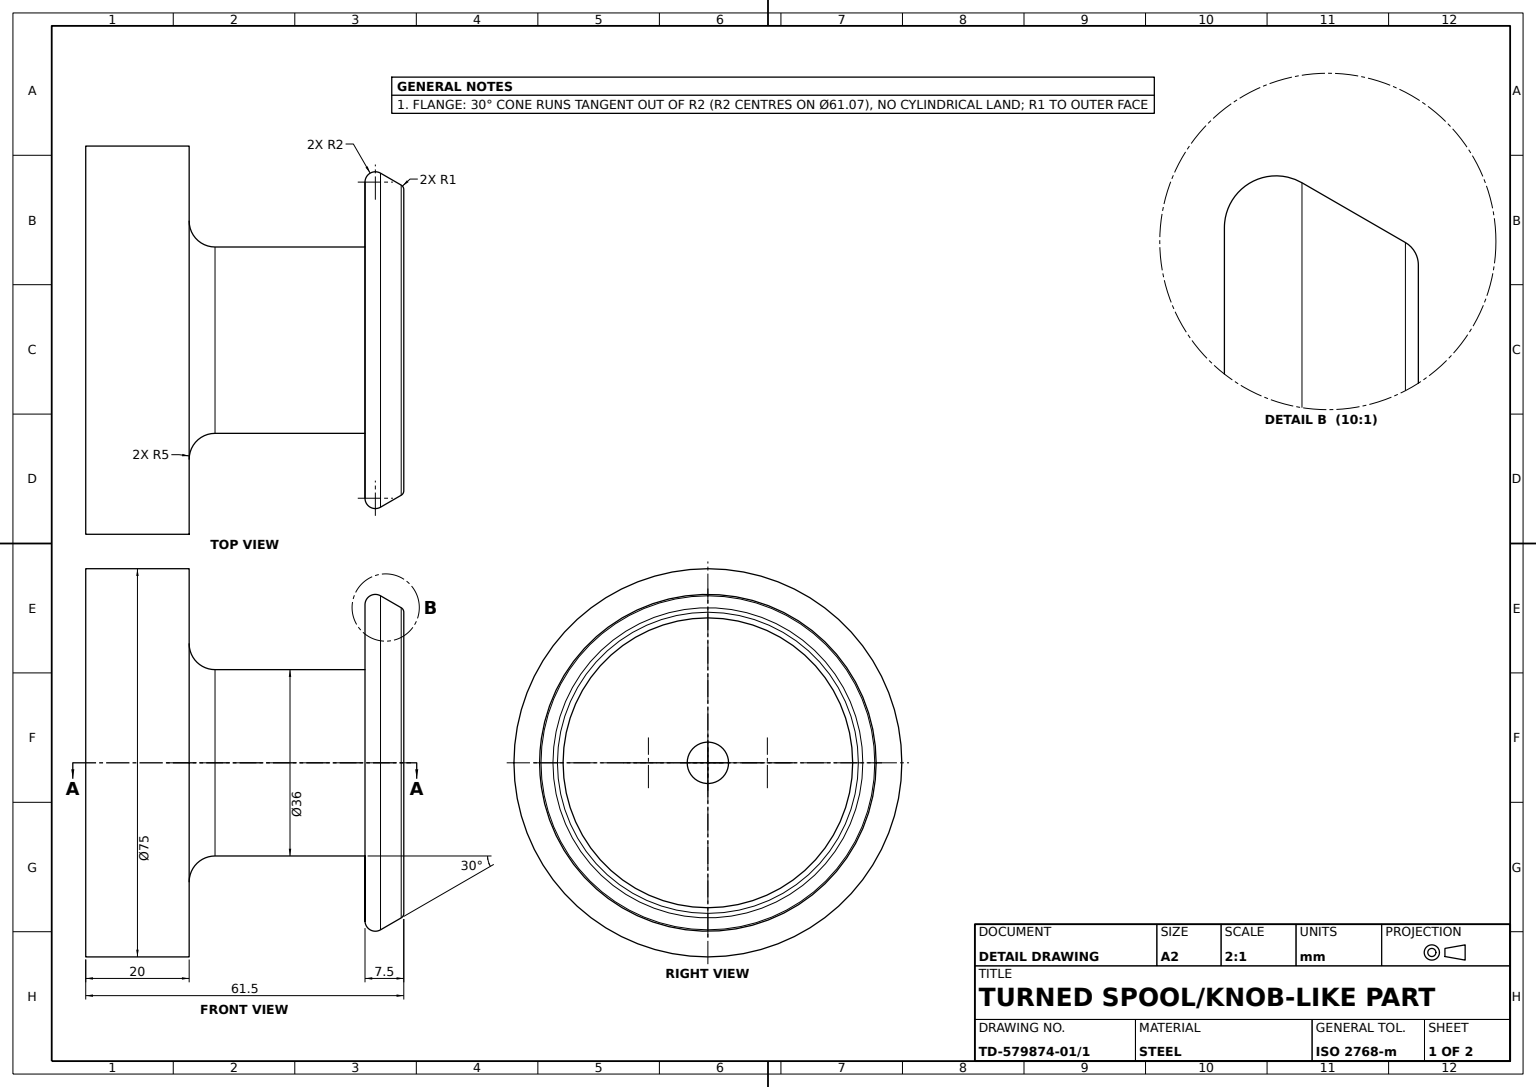
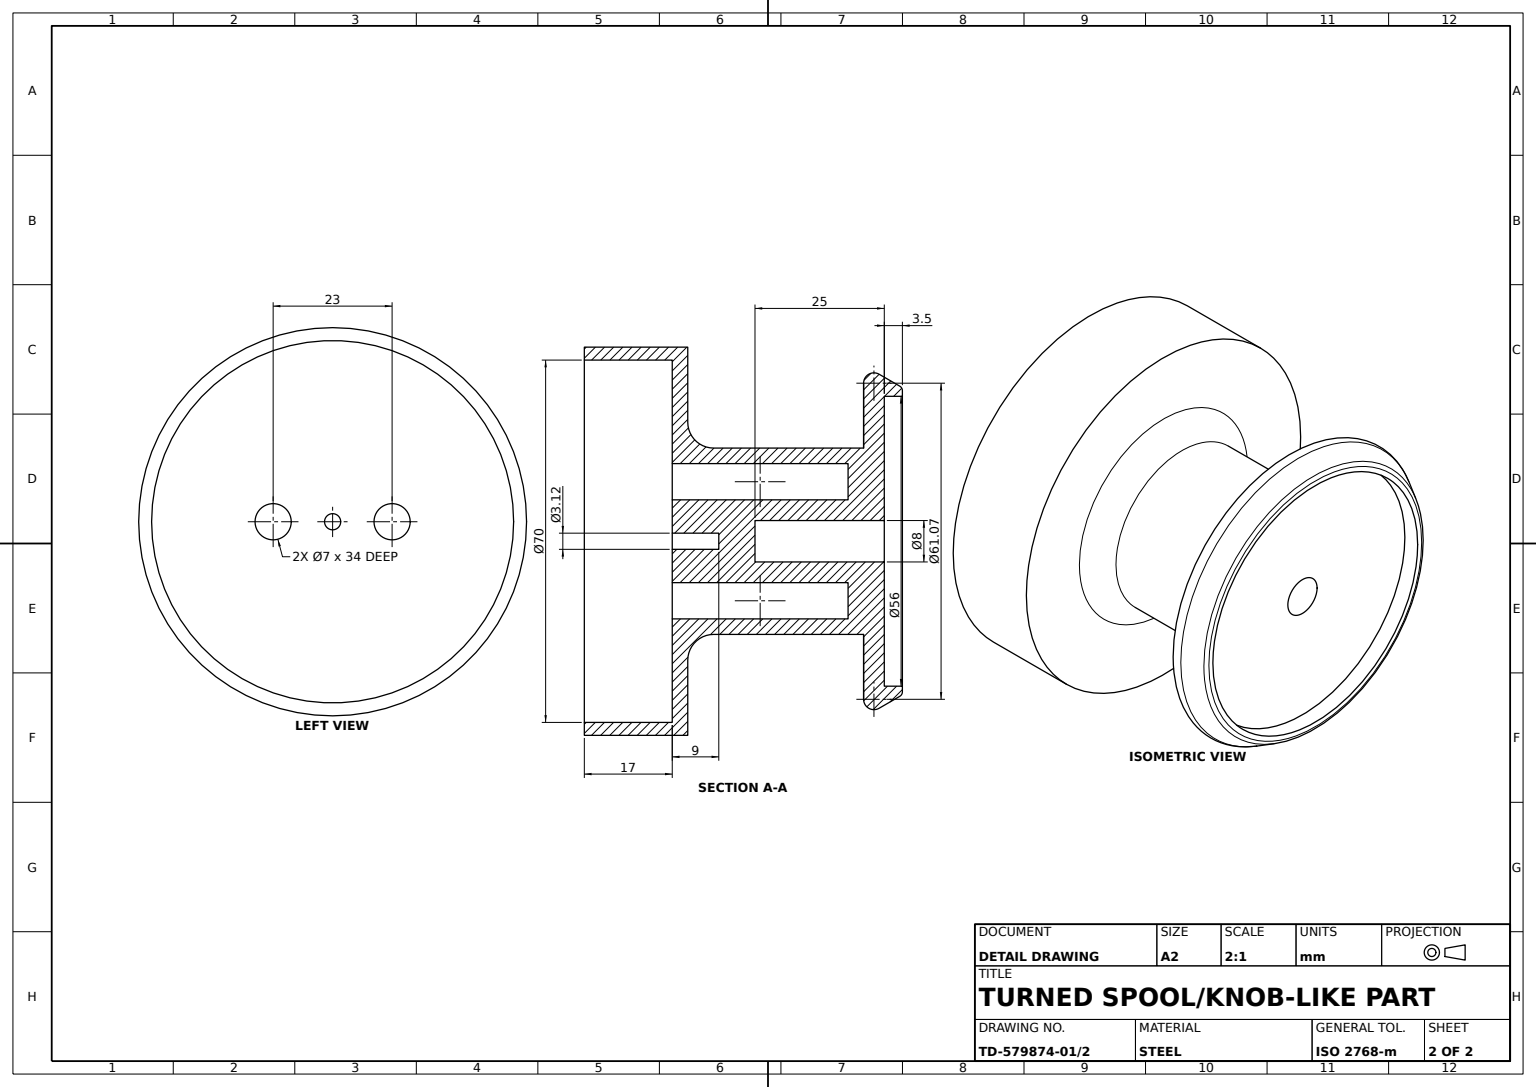
ISO-10303-21;
HEADER;
FILE_DESCRIPTION((''),'2;1');
FILE_NAME('','',(''),(''),'','','');
FILE_SCHEMA(('AUTOMOTIVE_DESIGN'));
ENDSEC;
DATA;
#1=APPLICATION_CONTEXT('');
#2=PRODUCT_CONTEXT('',#1,'mechanical');
#3=PRODUCT('','','',(#2));
#4=PRODUCT_DEFINITION_FORMATION('','',#3);
#5=PRODUCT_DEFINITION_CONTEXT('',#1,'design');
#6=PRODUCT_DEFINITION('','',#4,#5);
#7=PRODUCT_DEFINITION_SHAPE('','',#6);
#8=(LENGTH_UNIT()NAMED_UNIT(*)SI_UNIT(.MILLI.,.METRE.));
#9=(NAMED_UNIT(*)PLANE_ANGLE_UNIT()SI_UNIT($,.RADIAN.));
#10=(NAMED_UNIT(*)SI_UNIT($,.STERADIAN.)SOLID_ANGLE_UNIT());
#11=UNCERTAINTY_MEASURE_WITH_UNIT(LENGTH_MEASURE(1.E-05),#8,'distance_accuracy_value','');
#12=(GEOMETRIC_REPRESENTATION_CONTEXT(3)GLOBAL_UNCERTAINTY_ASSIGNED_CONTEXT((#11))GLOBAL_UNIT_ASSIGNED_CONTEXT((#8,#9,#10))REPRESENTATION_CONTEXT('',''));
#13=CARTESIAN_POINT('',(0.,61.5,29.092523));
#14=VERTEX_POINT('',#13);
#15=CARTESIAN_POINT('',(0.,61.5,-29.092523));
#16=VERTEX_POINT('',#15);
#17=CARTESIAN_POINT('',(0.,61.5,0.));
#18=DIRECTION('',(0.,1.,0.));
#19=DIRECTION('',(0.,0.,1.));
#20=AXIS2_PLACEMENT_3D('',#17,#18,#19);
#21=CIRCLE('',#20,29.092523);
#22=EDGE_CURVE('',#14,#16,#21,.T.);
#23=ORIENTED_EDGE('',*,*,#22,.T.);
#24=EDGE_CURVE('',#16,#14,#21,.T.);
#25=ORIENTED_EDGE('',*,*,#24,.T.);
#26=EDGE_LOOP('',(#23,#25));
#27=FACE_OUTER_BOUND('',#26,.T.);
#28=CARTESIAN_POINT('',(0.,61.5,-28.));
#29=VERTEX_POINT('',#28);
#30=CARTESIAN_POINT('',(0.,61.5,28.));
#31=VERTEX_POINT('',#30);
#32=CIRCLE('',#20,28.);
#33=EDGE_CURVE('',#29,#31,#32,.T.);
#34=ORIENTED_EDGE('',*,*,#33,.F.);
#35=EDGE_CURVE('',#31,#29,#32,.T.);
#36=ORIENTED_EDGE('',*,*,#35,.F.);
#37=EDGE_LOOP('',(#34,#36));
#38=FACE_BOUND('',#37,.T.);
#39=PLANE('',#20);
#40=ADVANCED_FACE('',(#27,#38),#39,.T.);
#41=CARTESIAN_POINT('',(0.,61.,29.958548));
#42=VERTEX_POINT('',#41);
#43=CARTESIAN_POINT('',(0.,61.,-29.958548));
#44=VERTEX_POINT('',#43);
#45=CARTESIAN_POINT('',(0.,61.,0.));
#46=DIRECTION('',(0.,-1.,0.));
#47=DIRECTION('',(0.,0.,-1.));
#48=AXIS2_PLACEMENT_3D('',#45,#46,#47);
#49=CIRCLE('',#48,29.958548);
#50=EDGE_CURVE('',#42,#44,#49,.T.);
#51=ORIENTED_EDGE('',*,*,#50,.F.);
#52=CARTESIAN_POINT('',(0.,60.5,29.092523));
#53=DIRECTION('',(-1.,0.,0.));
#54=AXIS2_PLACEMENT_3D('',#52,#53,#19);
#55=CIRCLE('',#54,1.);
#56=EDGE_CURVE('',#42,#14,#55,.T.);
#57=ORIENTED_EDGE('',*,*,#56,.T.);
#58=ORIENTED_EDGE('',*,*,#24,.F.);
#59=CARTESIAN_POINT('',(0.,60.5,-29.092523));
#60=DIRECTION('',(1.,0.,0.));
#61=AXIS2_PLACEMENT_3D('',#59,#60,#47);
#62=CIRCLE('',#61,1.);
#63=EDGE_CURVE('',#44,#16,#62,.T.);
#64=ORIENTED_EDGE('',*,*,#63,.F.);
#65=EDGE_LOOP('',(#51,#57,#58,#64));
#66=FACE_OUTER_BOUND('',#65,.T.);
#67=CARTESIAN_POINT('',(0.,60.5,0.));
#68=AXIS2_PLACEMENT_3D('',#67,#18,#19);
#69=TOROIDAL_SURFACE('',#68,29.092523,1.);
#70=ADVANCED_FACE('',(#66),#69,.T.);
#71=CARTESIAN_POINT('',(0.,51.,-15.));
#72=VERTEX_POINT('',#71);
#73=CARTESIAN_POINT('',(0.,17.,-15.));
#74=VERTEX_POINT('',#73);
#75=VECTOR('',#46,1000.);
#76=LINE('',#71,#75);
#77=EDGE_CURVE('',#72,#74,#76,.T.);
#78=ORIENTED_EDGE('',*,*,#77,.T.);
#79=CARTESIAN_POINT('',(0.,17.,-8.));
#80=VERTEX_POINT('',#79);
#81=CARTESIAN_POINT('',(0.,17.,-11.5));
#82=AXIS2_PLACEMENT_3D('',#81,#46,#47);
#83=CIRCLE('',#82,3.5);
#84=EDGE_CURVE('',#74,#80,#83,.T.);
#85=ORIENTED_EDGE('',*,*,#84,.T.);
#86=CARTESIAN_POINT('',(0.,51.,-8.));
#87=VERTEX_POINT('',#86);
#88=LINE('',#86,#75);
#89=EDGE_CURVE('',#87,#80,#88,.T.);
#90=ORIENTED_EDGE('',*,*,#89,.F.);
#91=CARTESIAN_POINT('',(0.,51.,-11.5));
#92=AXIS2_PLACEMENT_3D('',#91,#46,#47);
#93=CIRCLE('',#92,3.5);
#94=EDGE_CURVE('',#72,#87,#93,.T.);
#95=ORIENTED_EDGE('',*,*,#94,.F.);
#96=EDGE_LOOP('',(#78,#85,#90,#95));
#97=FACE_OUTER_BOUND('',#96,.T.);
#98=CYLINDRICAL_SURFACE('',#92,3.5);
#99=ADVANCED_FACE('',(#97),#98,.F.);
#100=EDGE_CURVE('',#44,#42,#49,.T.);
#101=ORIENTED_EDGE('',*,*,#100,.F.);
#102=ORIENTED_EDGE('',*,*,#63,.T.);
#103=ORIENTED_EDGE('',*,*,#22,.F.);
#104=ORIENTED_EDGE('',*,*,#56,.F.);
#105=EDGE_LOOP('',(#101,#102,#103,#104));
#106=FACE_OUTER_BOUND('',#105,.T.);
#107=ADVANCED_FACE('',(#106),#69,.T.);
#108=CARTESIAN_POINT('',(0.,20.,23.));
#109=VERTEX_POINT('',#108);
#110=CARTESIAN_POINT('',(0.,20.,-23.));
#111=VERTEX_POINT('',#110);
#112=CARTESIAN_POINT('',(0.,20.,0.));
#113=AXIS2_PLACEMENT_3D('',#112,#46,#19);
#114=CIRCLE('',#113,23.);
#115=EDGE_CURVE('',#109,#111,#114,.T.);
#116=ORIENTED_EDGE('',*,*,#115,.F.);
#117=CARTESIAN_POINT('',(0.,25.,18.));
#118=VERTEX_POINT('',#117);
#119=CARTESIAN_POINT('',(0.,25.,23.));
#120=AXIS2_PLACEMENT_3D('',#119,#53,#19);
#121=CIRCLE('',#120,5.);
#122=EDGE_CURVE('',#118,#109,#121,.T.);
#123=ORIENTED_EDGE('',*,*,#122,.F.);
#124=CARTESIAN_POINT('',(0.,25.,-18.));
#125=VERTEX_POINT('',#124);
#126=CARTESIAN_POINT('',(0.,25.,0.));
#127=AXIS2_PLACEMENT_3D('',#126,#18,#19);
#128=CIRCLE('',#127,18.);
#129=EDGE_CURVE('',#125,#118,#128,.T.);
#130=ORIENTED_EDGE('',*,*,#129,.F.);
#131=CARTESIAN_POINT('',(0.,25.,-23.));
#132=AXIS2_PLACEMENT_3D('',#131,#60,#47);
#133=CIRCLE('',#132,5.);
#134=EDGE_CURVE('',#125,#111,#133,.T.);
#135=ORIENTED_EDGE('',*,*,#134,.T.);
#136=EDGE_LOOP('',(#116,#123,#130,#135));
#137=FACE_OUTER_BOUND('',#136,.T.);
#138=TOROIDAL_SURFACE('',#127,23.,5.);
#139=ADVANCED_FACE('',(#137),#138,.F.);
#140=ORIENTED_EDGE('',*,*,#94,.T.);
#141=EDGE_CURVE('',#87,#72,#93,.T.);
#142=ORIENTED_EDGE('',*,*,#141,.T.);
#143=EDGE_LOOP('',(#140,#142));
#144=FACE_OUTER_BOUND('',#143,.T.);
#145=CARTESIAN_POINT('',(0.,51.,0.));
#146=AXIS2_PLACEMENT_3D('',#145,#46,#47);
#147=PLANE('',#146);
#148=ADVANCED_FACE('',(#144),#147,.T.);
#149=CARTESIAN_POINT('',(0.,17.,35.));
#150=VERTEX_POINT('',#149);
#151=CARTESIAN_POINT('',(0.,17.,-35.));
#152=VERTEX_POINT('',#151);
#153=CARTESIAN_POINT('',(0.,17.,0.));
#154=AXIS2_PLACEMENT_3D('',#153,#46,#47);
#155=CIRCLE('',#154,35.);
#156=EDGE_CURVE('',#150,#152,#155,.T.);
#157=ORIENTED_EDGE('',*,*,#156,.F.);
#158=CARTESIAN_POINT('',(0.,0.,35.));
#159=VERTEX_POINT('',#158);
#160=LINE('',#149,#75);
#161=EDGE_CURVE('',#150,#159,#160,.T.);
#162=ORIENTED_EDGE('',*,*,#161,.T.);
#163=CARTESIAN_POINT('',(0.,0.,-35.));
#164=VERTEX_POINT('',#163);
#165=CARTESIAN_POINT('',(0.,0.,0.));
#166=AXIS2_PLACEMENT_3D('',#165,#46,#47);
#167=CIRCLE('',#166,35.);
#168=EDGE_CURVE('',#159,#164,#167,.T.);
#169=ORIENTED_EDGE('',*,*,#168,.T.);
#170=LINE('',#151,#75);
#171=EDGE_CURVE('',#152,#164,#170,.T.);
#172=ORIENTED_EDGE('',*,*,#171,.F.);
#173=EDGE_LOOP('',(#157,#162,#169,#172));
#174=FACE_OUTER_BOUND('',#173,.T.);
#175=CYLINDRICAL_SURFACE('',#154,35.);
#176=ADVANCED_FACE('',(#174),#175,.F.);
#177=CARTESIAN_POINT('',(0.,58.,-28.));
#178=VERTEX_POINT('',#177);
#179=CARTESIAN_POINT('',(0.,58.,28.));
#180=VERTEX_POINT('',#179);
#181=CARTESIAN_POINT('',(0.,58.,0.));
#182=AXIS2_PLACEMENT_3D('',#181,#18,#19);
#183=CIRCLE('',#182,28.);
#184=EDGE_CURVE('',#178,#180,#183,.T.);
#185=ORIENTED_EDGE('',*,*,#184,.T.);
#186=EDGE_CURVE('',#180,#178,#183,.T.);
#187=ORIENTED_EDGE('',*,*,#186,.T.);
#188=EDGE_LOOP('',(#185,#187));
#189=FACE_OUTER_BOUND('',#188,.T.);
#190=CARTESIAN_POINT('',(0.,58.,-4.));
#191=VERTEX_POINT('',#190);
#192=CARTESIAN_POINT('',(0.,58.,4.));
#193=VERTEX_POINT('',#192);
#194=CIRCLE('',#182,4.);
#195=EDGE_CURVE('',#191,#193,#194,.T.);
#196=ORIENTED_EDGE('',*,*,#195,.F.);
#197=EDGE_CURVE('',#193,#191,#194,.T.);
#198=ORIENTED_EDGE('',*,*,#197,.F.);
#199=EDGE_LOOP('',(#196,#198));
#200=FACE_BOUND('',#199,.T.);
#201=PLANE('',#182);
#202=ADVANCED_FACE('',(#189,#200),#201,.T.);
#203=ORIENTED_EDGE('',*,*,#129,.T.);
#204=CARTESIAN_POINT('',(0.,54.,18.));
#205=VERTEX_POINT('',#204);
#206=LINE('',#204,#75);
#207=EDGE_CURVE('',#205,#118,#206,.T.);
#208=ORIENTED_EDGE('',*,*,#207,.F.);
#209=CARTESIAN_POINT('',(0.,54.,-18.));
#210=VERTEX_POINT('',#209);
#211=CARTESIAN_POINT('',(0.,54.,0.));
#212=AXIS2_PLACEMENT_3D('',#211,#18,#19);
#213=CIRCLE('',#212,18.);
#214=EDGE_CURVE('',#210,#205,#213,.T.);
#215=ORIENTED_EDGE('',*,*,#214,.F.);
#216=LINE('',#209,#75);
#217=EDGE_CURVE('',#210,#125,#216,.T.);
#218=ORIENTED_EDGE('',*,*,#217,.T.);
#219=EDGE_LOOP('',(#203,#208,#215,#218));
#220=FACE_OUTER_BOUND('',#219,.T.);
#221=AXIS2_PLACEMENT_3D('',#211,#46,#47);
#222=CYLINDRICAL_SURFACE('',#221,18.);
#223=ADVANCED_FACE('',(#220),#222,.T.);
#224=CARTESIAN_POINT('',(0.,17.,15.));
#225=VERTEX_POINT('',#224);
#226=CARTESIAN_POINT('',(0.,17.,8.));
#227=VERTEX_POINT('',#226);
#228=CARTESIAN_POINT('',(0.,17.,11.5));
#229=AXIS2_PLACEMENT_3D('',#228,#46,#47);
#230=CIRCLE('',#229,3.5);
#231=EDGE_CURVE('',#225,#227,#230,.T.);
#232=ORIENTED_EDGE('',*,*,#231,.T.);
#233=CARTESIAN_POINT('',(0.,51.,8.));
#234=VERTEX_POINT('',#233);
#235=LINE('',#233,#75);
#236=EDGE_CURVE('',#234,#227,#235,.T.);
#237=ORIENTED_EDGE('',*,*,#236,.F.);
#238=CARTESIAN_POINT('',(0.,51.,15.));
#239=VERTEX_POINT('',#238);
#240=CARTESIAN_POINT('',(0.,51.,11.5));
#241=AXIS2_PLACEMENT_3D('',#240,#46,#47);
#242=CIRCLE('',#241,3.5);
#243=EDGE_CURVE('',#239,#234,#242,.T.);
#244=ORIENTED_EDGE('',*,*,#243,.F.);
#245=LINE('',#238,#75);
#246=EDGE_CURVE('',#239,#225,#245,.T.);
#247=ORIENTED_EDGE('',*,*,#246,.T.);
#248=EDGE_LOOP('',(#232,#237,#244,#247));
#249=FACE_OUTER_BOUND('',#248,.T.);
#250=CYLINDRICAL_SURFACE('',#241,3.5);
#251=ADVANCED_FACE('',(#249),#250,.F.);
#252=CARTESIAN_POINT('',(0.,54.,-30.535898));
#253=VERTEX_POINT('',#252);
#254=CARTESIAN_POINT('',(0.,57.,-32.267949));
#255=VERTEX_POINT('',#254);
#256=CARTESIAN_POINT('',(0.,56.,-30.535898));
#257=AXIS2_PLACEMENT_3D('',#256,#60,#47);
#258=CIRCLE('',#257,2.);
#259=EDGE_CURVE('',#253,#255,#258,.T.);
#260=ORIENTED_EDGE('',*,*,#259,.F.);
#261=CARTESIAN_POINT('',(0.,54.,30.535898));
#262=VERTEX_POINT('',#261);
#263=AXIS2_PLACEMENT_3D('',#211,#46,#19);
#264=CIRCLE('',#263,30.535898);
#265=EDGE_CURVE('',#262,#253,#264,.T.);
#266=ORIENTED_EDGE('',*,*,#265,.F.);
#267=CARTESIAN_POINT('',(0.,57.,32.267949));
#268=VERTEX_POINT('',#267);
#269=CARTESIAN_POINT('',(0.,56.,30.535898));
#270=AXIS2_PLACEMENT_3D('',#269,#53,#19);
#271=CIRCLE('',#270,2.);
#272=EDGE_CURVE('',#262,#268,#271,.T.);
#273=ORIENTED_EDGE('',*,*,#272,.T.);
#274=CARTESIAN_POINT('',(0.,57.,0.));
#275=AXIS2_PLACEMENT_3D('',#274,#18,#19);
#276=CIRCLE('',#275,32.267949);
#277=EDGE_CURVE('',#255,#268,#276,.T.);
#278=ORIENTED_EDGE('',*,*,#277,.F.);
#279=EDGE_LOOP('',(#260,#266,#273,#278));
#280=FACE_OUTER_BOUND('',#279,.T.);
#281=CARTESIAN_POINT('',(0.,56.,0.));
#282=AXIS2_PLACEMENT_3D('',#281,#18,#19);
#283=TOROIDAL_SURFACE('',#282,30.535898,2.);
#284=ADVANCED_FACE('',(#280),#283,.T.);
#285=EDGE_CURVE('',#234,#239,#242,.T.);
#286=ORIENTED_EDGE('',*,*,#285,.T.);
#287=ORIENTED_EDGE('',*,*,#243,.T.);
#288=EDGE_LOOP('',(#286,#287));
#289=FACE_OUTER_BOUND('',#288,.T.);
#290=PLANE('',#241);
#291=ADVANCED_FACE('',(#289),#290,.T.);
#292=ORIENTED_EDGE('',*,*,#231,.F.);
#293=EDGE_CURVE('',#227,#225,#230,.T.);
#294=ORIENTED_EDGE('',*,*,#293,.F.);
#295=EDGE_LOOP('',(#292,#294));
#296=FACE_BOUND('',#295,.T.);
#297=EDGE_CURVE('',#80,#74,#83,.T.);
#298=ORIENTED_EDGE('',*,*,#297,.F.);
#299=ORIENTED_EDGE('',*,*,#84,.F.);
#300=EDGE_LOOP('',(#298,#299));
#301=FACE_BOUND('',#300,.T.);
#302=EDGE_CURVE('',#152,#150,#155,.T.);
#303=ORIENTED_EDGE('',*,*,#302,.T.);
#304=ORIENTED_EDGE('',*,*,#156,.T.);
#305=EDGE_LOOP('',(#303,#304));
#306=FACE_OUTER_BOUND('',#305,.T.);
#307=CARTESIAN_POINT('',(0.,17.,1.562112));
#308=VERTEX_POINT('',#307);
#309=CARTESIAN_POINT('',(0.,17.,-1.562112));
#310=VERTEX_POINT('',#309);
#311=CIRCLE('',#154,1.562112);
#312=EDGE_CURVE('',#308,#310,#311,.T.);
#313=ORIENTED_EDGE('',*,*,#312,.F.);
#314=EDGE_CURVE('',#310,#308,#311,.T.);
#315=ORIENTED_EDGE('',*,*,#314,.F.);
#316=EDGE_LOOP('',(#313,#315));
#317=FACE_BOUND('',#316,.T.);
#318=PLANE('',#154);
#319=ADVANCED_FACE('',(#296,#301,#306,#317),#318,.T.);
#320=ORIENTED_EDGE('',*,*,#161,.F.);
#321=ORIENTED_EDGE('',*,*,#302,.F.);
#322=ORIENTED_EDGE('',*,*,#171,.T.);
#323=EDGE_CURVE('',#164,#159,#167,.T.);
#324=ORIENTED_EDGE('',*,*,#323,.T.);
#325=EDGE_LOOP('',(#320,#321,#322,#324));
#326=FACE_OUTER_BOUND('',#325,.T.);
#327=ADVANCED_FACE('',(#326),#175,.F.);
#328=EDGE_CURVE('',#118,#125,#128,.T.);
#329=ORIENTED_EDGE('',*,*,#328,.T.);
#330=ORIENTED_EDGE('',*,*,#217,.F.);
#331=EDGE_CURVE('',#205,#210,#213,.T.);
#332=ORIENTED_EDGE('',*,*,#331,.F.);
#333=ORIENTED_EDGE('',*,*,#207,.T.);
#334=EDGE_LOOP('',(#329,#330,#332,#333));
#335=FACE_OUTER_BOUND('',#334,.T.);
#336=ADVANCED_FACE('',(#335),#222,.T.);
#337=ORIENTED_EDGE('',*,*,#272,.F.);
#338=EDGE_CURVE('',#253,#262,#264,.T.);
#339=ORIENTED_EDGE('',*,*,#338,.F.);
#340=ORIENTED_EDGE('',*,*,#259,.T.);
#341=EDGE_CURVE('',#268,#255,#276,.T.);
#342=ORIENTED_EDGE('',*,*,#341,.F.);
#343=EDGE_LOOP('',(#337,#339,#340,#342));
#344=FACE_OUTER_BOUND('',#343,.T.);
#345=ADVANCED_FACE('',(#344),#283,.T.);
#346=ORIENTED_EDGE('',*,*,#77,.F.);
#347=ORIENTED_EDGE('',*,*,#141,.F.);
#348=ORIENTED_EDGE('',*,*,#89,.T.);
#349=ORIENTED_EDGE('',*,*,#297,.T.);
#350=EDGE_LOOP('',(#346,#347,#348,#349));
#351=FACE_OUTER_BOUND('',#350,.T.);
#352=ADVANCED_FACE('',(#351),#98,.F.);
#353=CARTESIAN_POINT('',(0.,33.,4.));
#354=VERTEX_POINT('',#353);
#355=CARTESIAN_POINT('',(0.,33.,-4.));
#356=VERTEX_POINT('',#355);
#357=CARTESIAN_POINT('',(0.,33.,0.));
#358=AXIS2_PLACEMENT_3D('',#357,#18,#19);
#359=CIRCLE('',#358,4.);
#360=EDGE_CURVE('',#354,#356,#359,.T.);
#361=ORIENTED_EDGE('',*,*,#360,.T.);
#362=EDGE_CURVE('',#356,#354,#359,.T.);
#363=ORIENTED_EDGE('',*,*,#362,.T.);
#364=EDGE_LOOP('',(#361,#363));
#365=FACE_OUTER_BOUND('',#364,.T.);
#366=PLANE('',#358);
#367=ADVANCED_FACE('',(#365),#366,.T.);
#368=CARTESIAN_POINT('',(0.,26.,1.562112));
#369=VERTEX_POINT('',#368);
#370=CARTESIAN_POINT('',(0.,26.,-1.562112));
#371=VERTEX_POINT('',#370);
#372=CARTESIAN_POINT('',(0.,26.,0.));
#373=AXIS2_PLACEMENT_3D('',#372,#46,#47);
#374=CIRCLE('',#373,1.562112);
#375=EDGE_CURVE('',#369,#371,#374,.T.);
#376=ORIENTED_EDGE('',*,*,#375,.T.);
#377=EDGE_CURVE('',#371,#369,#374,.T.);
#378=ORIENTED_EDGE('',*,*,#377,.T.);
#379=EDGE_LOOP('',(#376,#378));
#380=FACE_OUTER_BOUND('',#379,.T.);
#381=PLANE('',#373);
#382=ADVANCED_FACE('',(#380),#381,.T.);
#383=ORIENTED_EDGE('',*,*,#362,.F.);
#384=VECTOR('',#18,1000.);
#385=LINE('',#355,#384);
#386=EDGE_CURVE('',#356,#191,#385,.T.);
#387=ORIENTED_EDGE('',*,*,#386,.T.);
#388=ORIENTED_EDGE('',*,*,#195,.T.);
#389=LINE('',#353,#384);
#390=EDGE_CURVE('',#354,#193,#389,.T.);
#391=ORIENTED_EDGE('',*,*,#390,.F.);
#392=EDGE_LOOP('',(#383,#387,#388,#391));
#393=FACE_OUTER_BOUND('',#392,.T.);
#394=CYLINDRICAL_SURFACE('',#358,4.);
#395=ADVANCED_FACE('',(#393),#394,.F.);
#396=CARTESIAN_POINT('',(0.,20.,-37.5));
#397=VERTEX_POINT('',#396);
#398=CARTESIAN_POINT('',(0.,20.,37.5));
#399=VERTEX_POINT('',#398);
#400=AXIS2_PLACEMENT_3D('',#112,#18,#19);
#401=CIRCLE('',#400,37.5);
#402=EDGE_CURVE('',#397,#399,#401,.T.);
#403=ORIENTED_EDGE('',*,*,#402,.F.);
#404=CARTESIAN_POINT('',(0.,0.,-37.5));
#405=VERTEX_POINT('',#404);
#406=LINE('',#396,#75);
#407=EDGE_CURVE('',#397,#405,#406,.T.);
#408=ORIENTED_EDGE('',*,*,#407,.T.);
#409=CARTESIAN_POINT('',(0.,0.,37.5));
#410=VERTEX_POINT('',#409);
#411=AXIS2_PLACEMENT_3D('',#165,#18,#19);
#412=CIRCLE('',#411,37.5);
#413=EDGE_CURVE('',#405,#410,#412,.T.);
#414=ORIENTED_EDGE('',*,*,#413,.T.);
#415=LINE('',#398,#75);
#416=EDGE_CURVE('',#399,#410,#415,.T.);
#417=ORIENTED_EDGE('',*,*,#416,.F.);
#418=EDGE_LOOP('',(#403,#408,#414,#417));
#419=FACE_OUTER_BOUND('',#418,.T.);
#420=AXIS2_PLACEMENT_3D('',#112,#46,#47);
#421=CYLINDRICAL_SURFACE('',#420,37.5);
#422=ADVANCED_FACE('',(#419),#421,.T.);
#423=ORIENTED_EDGE('',*,*,#214,.T.);
#424=ORIENTED_EDGE('',*,*,#331,.T.);
#425=EDGE_LOOP('',(#423,#424));
#426=FACE_BOUND('',#425,.T.);
#427=ORIENTED_EDGE('',*,*,#265,.T.);
#428=ORIENTED_EDGE('',*,*,#338,.T.);
#429=EDGE_LOOP('',(#427,#428));
#430=FACE_OUTER_BOUND('',#429,.T.);
#431=PLANE('',#212);
#432=ADVANCED_FACE('',(#426,#430),#431,.F.);
#433=ORIENTED_EDGE('',*,*,#35,.T.);
#434=LINE('',#177,#384);
#435=EDGE_CURVE('',#178,#29,#434,.T.);
#436=ORIENTED_EDGE('',*,*,#435,.F.);
#437=ORIENTED_EDGE('',*,*,#186,.F.);
#438=LINE('',#179,#384);
#439=EDGE_CURVE('',#180,#31,#438,.T.);
#440=ORIENTED_EDGE('',*,*,#439,.T.);
#441=EDGE_LOOP('',(#433,#436,#437,#440));
#442=FACE_OUTER_BOUND('',#441,.T.);
#443=CYLINDRICAL_SURFACE('',#182,28.);
#444=ADVANCED_FACE('',(#442),#443,.F.);
#445=CARTESIAN_POINT('',(0.,54.,-34.));
#446=DIRECTION('',(0.,-0.866025404,-0.5));
#447=VECTOR('',#446,1000.);
#448=LINE('',#445,#447);
#449=EDGE_CURVE('',#44,#255,#448,.T.);
#450=ORIENTED_EDGE('',*,*,#449,.T.);
#451=ORIENTED_EDGE('',*,*,#277,.T.);
#452=CARTESIAN_POINT('',(0.,54.,34.));
#453=DIRECTION('',(0.,-0.866025404,0.5));
#454=VECTOR('',#453,1000.);
#455=LINE('',#452,#454);
#456=EDGE_CURVE('',#42,#268,#455,.T.);
#457=ORIENTED_EDGE('',*,*,#456,.F.);
#458=ORIENTED_EDGE('',*,*,#50,.T.);
#459=EDGE_LOOP('',(#450,#451,#457,#458));
#460=FACE_OUTER_BOUND('',#459,.T.);
#461=CONICAL_SURFACE('',#263,34.,0.523598776);
#462=ADVANCED_FACE('',(#460),#461,.T.);
#463=ORIENTED_EDGE('',*,*,#134,.F.);
#464=ORIENTED_EDGE('',*,*,#328,.F.);
#465=ORIENTED_EDGE('',*,*,#122,.T.);
#466=EDGE_CURVE('',#111,#109,#114,.T.);
#467=ORIENTED_EDGE('',*,*,#466,.F.);
#468=EDGE_LOOP('',(#463,#464,#465,#467));
#469=FACE_OUTER_BOUND('',#468,.T.);
#470=ADVANCED_FACE('',(#469),#138,.F.);
#471=ORIENTED_EDGE('',*,*,#377,.F.);
#472=LINE('',#370,#75);
#473=EDGE_CURVE('',#371,#310,#472,.T.);
#474=ORIENTED_EDGE('',*,*,#473,.T.);
#475=ORIENTED_EDGE('',*,*,#314,.T.);
#476=LINE('',#368,#75);
#477=EDGE_CURVE('',#369,#308,#476,.T.);
#478=ORIENTED_EDGE('',*,*,#477,.F.);
#479=EDGE_LOOP('',(#471,#474,#475,#478));
#480=FACE_OUTER_BOUND('',#479,.T.);
#481=CYLINDRICAL_SURFACE('',#373,1.562112);
#482=ADVANCED_FACE('',(#480),#481,.F.);
#483=ORIENTED_EDGE('',*,*,#360,.F.);
#484=ORIENTED_EDGE('',*,*,#390,.T.);
#485=ORIENTED_EDGE('',*,*,#197,.T.);
#486=ORIENTED_EDGE('',*,*,#386,.F.);
#487=EDGE_LOOP('',(#483,#484,#485,#486));
#488=FACE_OUTER_BOUND('',#487,.T.);
#489=ADVANCED_FACE('',(#488),#394,.F.);
#490=ORIENTED_EDGE('',*,*,#312,.T.);
#491=ORIENTED_EDGE('',*,*,#473,.F.);
#492=ORIENTED_EDGE('',*,*,#375,.F.);
#493=ORIENTED_EDGE('',*,*,#477,.T.);
#494=EDGE_LOOP('',(#490,#491,#492,#493));
#495=FACE_OUTER_BOUND('',#494,.T.);
#496=ADVANCED_FACE('',(#495),#481,.F.);
#497=ORIENTED_EDGE('',*,*,#407,.F.);
#498=EDGE_CURVE('',#399,#397,#401,.T.);
#499=ORIENTED_EDGE('',*,*,#498,.F.);
#500=ORIENTED_EDGE('',*,*,#416,.T.);
#501=EDGE_CURVE('',#410,#405,#412,.T.);
#502=ORIENTED_EDGE('',*,*,#501,.T.);
#503=EDGE_LOOP('',(#497,#499,#500,#502));
#504=FACE_OUTER_BOUND('',#503,.T.);
#505=ADVANCED_FACE('',(#504),#421,.T.);
#506=ORIENTED_EDGE('',*,*,#323,.F.);
#507=ORIENTED_EDGE('',*,*,#168,.F.);
#508=EDGE_LOOP('',(#506,#507));
#509=FACE_BOUND('',#508,.T.);
#510=ORIENTED_EDGE('',*,*,#501,.F.);
#511=ORIENTED_EDGE('',*,*,#413,.F.);
#512=EDGE_LOOP('',(#510,#511));
#513=FACE_OUTER_BOUND('',#512,.T.);
#514=PLANE('',#411);
#515=ADVANCED_FACE('',(#509,#513),#514,.F.);
#516=ORIENTED_EDGE('',*,*,#456,.T.);
#517=ORIENTED_EDGE('',*,*,#341,.T.);
#518=ORIENTED_EDGE('',*,*,#449,.F.);
#519=ORIENTED_EDGE('',*,*,#100,.T.);
#520=EDGE_LOOP('',(#516,#517,#518,#519));
#521=FACE_OUTER_BOUND('',#520,.T.);
#522=ADVANCED_FACE('',(#521),#461,.T.);
#523=ORIENTED_EDGE('',*,*,#115,.T.);
#524=ORIENTED_EDGE('',*,*,#466,.T.);
#525=EDGE_LOOP('',(#523,#524));
#526=FACE_BOUND('',#525,.T.);
#527=ORIENTED_EDGE('',*,*,#402,.T.);
#528=ORIENTED_EDGE('',*,*,#498,.T.);
#529=EDGE_LOOP('',(#527,#528));
#530=FACE_OUTER_BOUND('',#529,.T.);
#531=PLANE('',#400);
#532=ADVANCED_FACE('',(#526,#530),#531,.T.);
#533=ORIENTED_EDGE('',*,*,#285,.F.);
#534=ORIENTED_EDGE('',*,*,#236,.T.);
#535=ORIENTED_EDGE('',*,*,#293,.T.);
#536=ORIENTED_EDGE('',*,*,#246,.F.);
#537=EDGE_LOOP('',(#533,#534,#535,#536));
#538=FACE_OUTER_BOUND('',#537,.T.);
#539=ADVANCED_FACE('',(#538),#250,.F.);
#540=ORIENTED_EDGE('',*,*,#33,.T.);
#541=ORIENTED_EDGE('',*,*,#439,.F.);
#542=ORIENTED_EDGE('',*,*,#184,.F.);
#543=ORIENTED_EDGE('',*,*,#435,.T.);
#544=EDGE_LOOP('',(#540,#541,#542,#543));
#545=FACE_OUTER_BOUND('',#544,.T.);
#546=ADVANCED_FACE('',(#545),#443,.F.);
#547=CLOSED_SHELL('',(#40,#70,#99,#107,#139,#148,#176,#202,#223,#251,#284,#291,#319,#327,#336,#345,#352,#367,#382,#395,#422,#432,#444,#462,#470,#482,#489,#496,#505,#515,#522,#532,#539,#546));
#548=MANIFOLD_SOLID_BREP('',#547);
#549=ADVANCED_BREP_SHAPE_REPRESENTATION('',(#548),#12);
#550=SHAPE_DEFINITION_REPRESENTATION(#7,#549);
ENDSEC;
END-ISO-10303-21;
